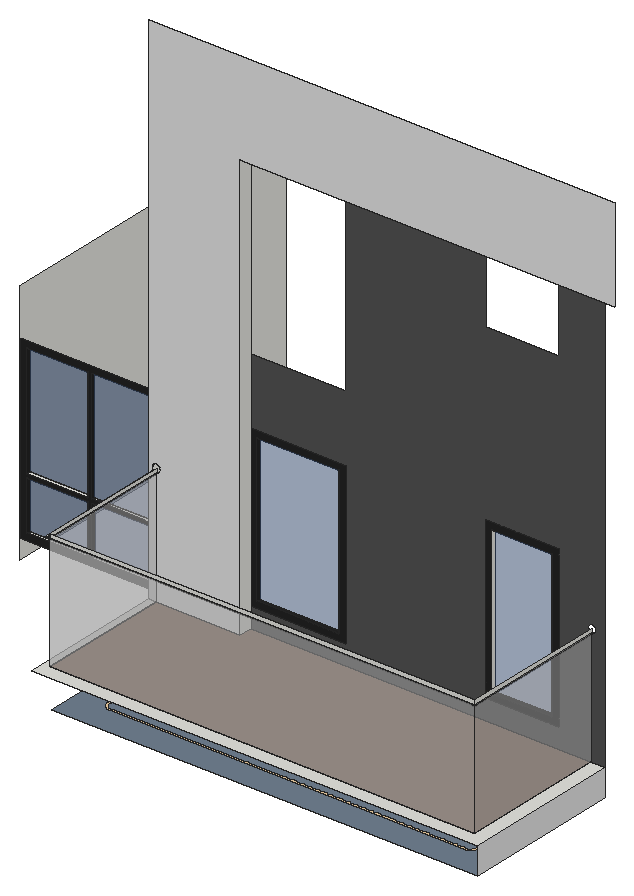
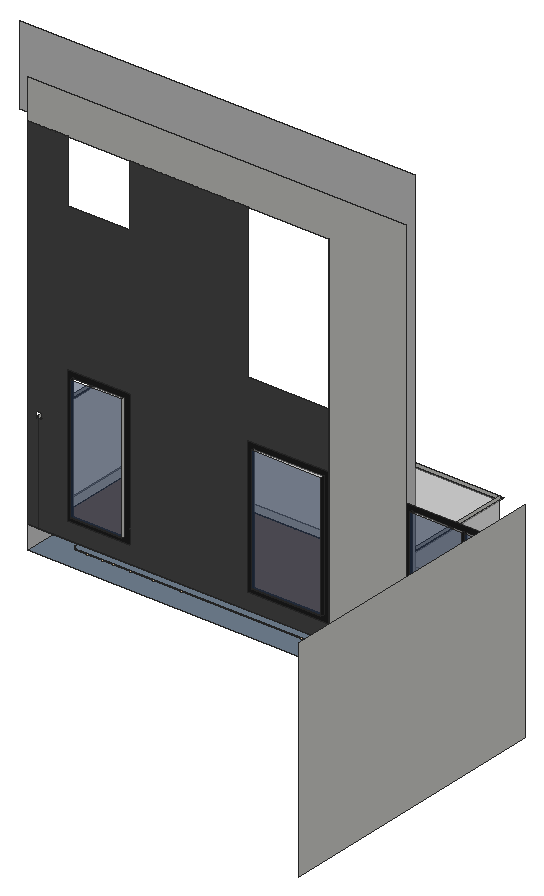
# SketchUp Ruby script. Lengths in inches.
U = 1.inch
M = Sketchup.active_model
def pt(a) = Geom::Point3d.new(a.map { |v| v * U })
def face(e, loops, mat)
  f = e.add_face(loops[0].map { |a| pt(a) })
  loops[1..].each { |l| e.add_face(l.map { |a| pt(a) }).erase! }
  f.material = f.back_material = mat if mat
  f
end
# faces: each face lists its corners as indices into pts; further lists are holes
def faces(e, pts, list, mat = nil) = list.each { |f| face(e, (f[0].is_a?(Array) ? f : [f]).map { |l| l.map { |i| pts[i] } }, mat) }
# xy, xz, yz: faces in a plane at the given z, y or x. An outline is a flat list of corners, or four numbers for a rectangle; further outlines are holes
def ring(l) = l.size == 4 ? [[l[0], l[1]], [l[2], l[1]], [l[2], l[3]], [l[0], l[3]]] : l.each_slice(2).to_a
def flat(e, list, mat, &to3) = list.each { |f| face(e, (f[0].is_a?(Array) ? f : [f]).map { |l| ring(l).map { |u, v| to3.(u, v) } }, mat) }
def xy(e, z, list, mat = nil) = flat(e, list, mat) { |x, y| [x, y, z] }
def xz(e, y, list, mat = nil) = flat(e, list, mat) { |x, z| [x, y, z] }
def yz(e, x, list, mat = nil) = flat(e, list, mat) { |y, z| [x, y, z] }
def lines(e, pts, list) = list.each { |a, b| e.add_line(pt(pts[a]), pt(pts[b])) }
# prism: a flat outline (further loops are holes) pulled along v
def prism(e, loops, v, mat = nil)
  f = face(e, loops, mat); d = Geom::Vector3d.new(v.map { |x| x * U })
  f.pushpull(f.normal.samedirection?(d) ? d.length : -d.length)
end
def box(e, o, s, mat = nil) = prism(e, [[o, [o[0] + s[0], o[1], o[2]], [o[0] + s[0], o[1] + s[1], o[2]], [o[0], o[1] + s[1], o[2]]]], [0, 0, s[2]], mat)
def at(x, y, z, deg = 0) = Geom::Transformation.translation(pt([x, y, z])) * Geom::Transformation.rotation(ORIGIN, Z_AXIS, deg.degrees)
def axes(o, x, y, z) = Geom::Transformation.new([*x, 0, *y, 0, *z, 0, *pt(o).to_a, 1])
def part(name) = M.definitions.add(name)
# library, detail: a bought-in or finely detailed component or shape, given as its bounding box
def library(name, o, s) = part(name).tap { |d| box(d.entities, o, s) }
def detail(e, o, s) = box(e.add_group.entities, o, s)
def put(e, d, t, mat = nil) = e.add_instance(d, t).tap { |i| i.material = mat if mat }
def group(e, t, mat = nil) = e.add_group.tap { |g| g.transformation = t; g.material = mat if mat }.entities
root = M.entities
M.materials.add("[0033_NavajoWhite]1").color = [237, 206, 160]
M.materials.add("[0111_SlateGray]").color = [112, 128, 144]
M.materials.add("[0136_Charcoal]").color = [35, 35, 35]
M.materials.add("[Cladding Siding White]1").color = [224, 224, 224]
M.materials.add("[Cladding Siding White]2").color = [81, 81, 81]
M.materials.add("[Granite Brown]").color = [126, 104, 91]
M.materials.add("[Translucent Glass Blue]").color = [52, 78, 124]
M.materials["[Translucent Glass Blue]"].alpha = 0.5
M.materials.add("[Translucent Glass Gray]").color = [211, 211, 211]
M.materials["[Translucent Glass Gray]"].alpha = 0.5
xy(root,1366.34,[[[412.89,49.29,410.86,49.43,408.86,49.83,406.92,50.48,405.09,51.38,403.4,52.52,401.86,53.86,400.52,55.4,399.38,57.09,398.48,58.92,397.83,60.86,397.43,62.86,397.29,64.89,397.29,223.11,397.43,225.14,397.83,227.14,398.48,229.08,399.38,230.91,400.52,232.6,401.86,234.14,403.4,235.48,405.09,236.62,406.92,237.52,408.86,238.17,410.86,238.57,412.89,238.71,1051.11,238.71,1053.14,238.57,1055.14,238.17,1057.08,237.52,1058.91,236.62,1060.6,235.48,1062.14,234.14,1063.48,232.6,1064.62,230.91,1065.52,229.08,1066.17,227.14,1066.57,225.14,1066.71,223.11,1066.71,64.89,1066.57,62.86,1066.17,60.86,1065.52,58.92,1064.62,57.09,1063.48,55.4,1062.14,53.86,1060.6,52.52,1058.91,51.38,1057.08,50.48,1055.14,49.83,1053.14,49.43,1051.11,49.29],[412.89,53.53,1051.11,53.53,1052.59,53.625,1054.05,53.92,1055.45,54.39,1056.79,55.05,1058.02,55.88,1059.14,56.86,1060.12,57.98,1060.95,59.21,1061.61,60.55,1062.08,61.95,1062.375,63.41,1062.47,64.89,1062.47,223.11,1062.375,224.59,1062.08,226.05,1061.61,227.45,1060.95,228.79,1060.12,230.02,1059.14,231.14,1058.02,232.12,1056.79,232.95,1055.45,233.61,1054.05,234.08,1052.59,234.375,1051.11,234.47,412.89,234.47,411.41,234.375,409.95,234.08,408.55,233.61,407.21,232.95,405.98,232.12,404.86,231.14,403.88,230.02,403.05,228.79,402.39,227.45,401.92,226.05,401.625,224.59,401.53,223.11,401.53,64.89,401.625,63.41,401.92,61.95,402.39,60.55,403.05,59.21,403.88,57.98,404.86,56.86,405.98,55.88,407.21,55.05,408.55,54.39,409.95,53.92,411.41,53.625]]],"[0033_NavajoWhite]1")
xy(root,1366.34,[[[348,0,1116,288],[412.89,49.29,1051.11,49.29,1053.14,49.43,1055.14,49.83,1057.08,50.48,1058.91,51.38,1060.6,52.52,1062.14,53.86,1063.48,55.4,1064.62,57.09,1065.52,58.92,1066.17,60.86,1066.57,62.86,1066.71,64.89,1066.71,223.11,1066.57,225.14,1066.17,227.14,1065.52,229.08,1064.62,230.91,1063.48,232.6,1062.14,234.14,1060.6,235.48,1058.91,236.62,1057.08,237.52,1055.14,238.17,1053.14,238.57,1051.11,238.71,412.89,238.71,410.86,238.57,408.86,238.17,406.92,237.52,405.09,236.62,403.4,235.48,401.86,234.14,400.52,232.6,399.38,230.91,398.48,229.08,397.83,227.14,397.43,225.14,397.29,223.11,397.29,64.89,397.43,62.86,397.83,60.86,398.48,58.92,399.38,57.09,400.52,55.4,401.86,53.86,403.4,52.52,405.09,51.38,406.92,50.48,408.86,49.83,410.86,49.43]],[[412.89,53.53,411.41,53.625,409.95,53.92,408.55,54.39,407.21,55.05,405.98,55.88,404.86,56.86,403.88,57.98,403.05,59.21,402.39,60.55,401.92,61.95,401.625,63.41,401.53,64.89,401.53,223.11,401.625,224.59,401.92,226.05,402.39,227.45,403.05,228.79,403.88,230.02,404.86,231.14,405.98,232.12,407.21,232.95,408.55,233.61,409.95,234.08,411.41,234.375,412.89,234.47,1051.11,234.47,1052.59,234.375,1054.05,234.08,1055.45,233.61,1056.79,232.95,1058.02,232.12,1059.14,231.14,1060.12,230.02,1060.95,228.79,1061.61,227.45,1062.08,226.05,1062.375,224.59,1062.47,223.11,1062.47,64.89,1062.375,63.41,1062.08,61.95,1061.61,60.55,1060.95,59.21,1060.12,57.98,1059.14,56.86,1058.02,55.88,1056.79,55.05,1055.45,54.39,1054.05,53.92,1052.59,53.625,1051.11,53.53],[535.65,130.71,536.9,130.83,538.13,131.08,539.33,131.46,540.48,131.96,541.58,132.58,542.6,133.32,543.54,134.15,544.38,135.08,545.13,136.09,545.77,137.17,546.29,138.3125,546.68,139.5,546.95,140.73,547.09,141.98,547.1,143.24,546.98,144.49,546.73,145.72,546.35,146.91,545.85,148.06,545.23,149.16,544.5,150.18,543.66,151.12,542.74,151.97,541.73,152.71,540.64,153.35,539.5,153.87,538.31,154.26,537.08,154.54,535.83,154.68,534.58,154.6875,533.33,154.5625,532.1,154.3125,530.9,153.93,529.75,153.43,528.66,152.8125,527.63,152.08,526.69,151.25,525.85,150.32,525.1,149.31,524.47,148.23,523.95,147.08,523.55,145.89,523.28,144.66,523.14,143.42,523.13,142.16,523.25,140.91,523.5,139.68,523.88,138.48,524.38,137.33,525,136.24,525.73,135.22,526.57,134.28,527.49,133.43,528.5,132.68,529.59,132.05,530.73,131.53,531.92,131.13,533.15,130.86,534.4,130.72],[899.19,130.71,900.44,130.83,901.67,131.08,902.86,131.46,904.01,131.96,905.11,132.58,906.13,133.32,907.07,134.15,907.92,135.08,908.66,136.09,909.3,137.17,909.82,138.3125,910.21,139.5,910.49,140.73,910.625,141.98,910.64,143.24,910.51,144.49,910.26,145.72,909.88,146.91,909.38,148.06,908.76,149.16,908.03,150.18,907.2,151.12,906.27,151.97,905.26,152.71,904.18,153.35,903.03,153.87,901.84,154.26,900.61,154.54,899.37,154.68,898.11,154.6875,896.86,154.5625,895.63,154.3125,894.43,153.93,893.28,153.43,892.1875,152.8125,891.17,152.08,890.23,151.25,889.38,150.32,888.63,149.31,888,148.23,887.48,147.08,887.08,145.89,886.81,144.66,886.67,143.42,886.66,142.16,886.78,140.91,887.03,139.68,887.41,138.48,887.91,137.33,888.53,136.24,889.27,135.22,890.1,134.28,891.03,133.43,892.04,132.68,893.12,132.05,894.26,131.53,895.45,131.13,896.68,130.86,897.93,130.72]]],"[0111_SlateGray]")
xy(root,1367.34,[[535.65,130.71,534.4,130.72,533.15,130.86,531.92,131.13,530.73,131.53,529.59,132.05,528.5,132.68,527.49,133.43,526.57,134.28,525.73,135.22,525,136.24,524.38,137.33,523.88,138.48,523.5,139.68,523.25,140.91,523.13,142.16,523.14,143.42,523.28,144.66,523.55,145.89,523.95,147.08,524.47,148.23,525.1,149.31,525.85,150.32,526.69,151.25,527.63,152.08,528.66,152.8125,529.75,153.43,530.9,153.93,532.1,154.3125,533.33,154.5625,534.58,154.6875,535.83,154.68,537.08,154.54,538.31,154.26,539.5,153.87,540.64,153.35,541.73,152.71,542.74,151.97,543.66,151.12,544.5,150.18,545.23,149.16,545.85,148.06,546.35,146.91,546.73,145.72,546.98,144.49,547.1,143.24,547.09,141.98,546.95,140.73,546.68,139.5,546.29,138.3125,545.77,137.17,545.13,136.09,544.38,135.08,543.54,134.15,542.6,133.32,541.58,132.58,540.48,131.96,539.33,131.46,538.13,131.08,536.9,130.83],[899.19,130.71,897.93,130.72,896.68,130.86,895.45,131.13,894.26,131.53,893.12,132.05,892.04,132.68,891.03,133.43,890.1,134.28,889.27,135.22,888.53,136.24,887.91,137.33,887.41,138.48,887.03,139.68,886.78,140.91,886.66,142.16,886.67,143.42,886.81,144.66,887.08,145.89,887.48,147.08,888,148.23,888.63,149.31,889.38,150.32,890.23,151.25,891.17,152.08,892.1875,152.8125,893.28,153.43,894.43,153.93,895.63,154.3125,896.86,154.5625,898.11,154.6875,899.37,154.68,900.61,154.54,901.84,154.26,903.03,153.87,904.18,153.35,905.26,152.71,906.27,151.97,907.2,151.12,908.03,150.18,908.76,149.16,909.38,148.06,909.88,146.91,910.26,145.72,910.51,144.49,910.64,143.24,910.625,141.98,910.49,140.73,910.21,139.5,909.82,138.3125,909.3,137.17,908.66,136.09,907.92,135.08,907.07,134.15,906.13,133.32,905.11,132.58,904.01,131.96,902.86,131.46,901.67,131.08,900.44,130.83]])
xy(root,1416,[[312,0,1116,0,1116,288,1092.15,288,1092.15,24,325.23,24,325.23,264,312,264]])
xy(root,1416,[[325.23,24,1092.15,24,1092.15,288,475.9375,288,475.9375,264,325.23,264]],"[Granite Brown]")
xy(root,1428,[[72,288,183,294],[189,288,300,295]])
xy(root,1464,[[487.9375,288,636,294],[912,288,1020,294]],"[0136_Charcoal]")
xy(root,1518,[[72,288,183,294],[189,288,300,295]],"[0136_Charcoal]")
xy(root,1524,[[72,288,183,294],[189,288,300,294]])
xz(root,24,[[325.23,1625,1092.15,1632]])
xz(root,24,[[325.23,1416,1092.15,1625]],"[Translucent Glass Gray]")
xz(root,264,[[325.23,1625,324.5,1625.04,323.78,1625.15,323.07,1625.34,322.39,1625.61,321.73,1625.9375,321.12,1626.34,320.55,1626.8,320.03,1627.32,319.57,1627.89,319.17,1628.5,318.84,1629.15,318.58,1629.84,318.39,1630.54,318.27,1631.27,318.23,1632,318.27,1632.73,318.39,1633.46,318.58,1634.16,318.84,1634.85,319.17,1635.5,319.57,1636.11,320.03,1636.68,320.55,1637.2,321.12,1637.66,321.73,1638.0625,322.39,1638.39,323.07,1638.66,323.78,1638.85,324.5,1638.96,325.23,1639,325.96,1638.96,326.6875,1638.85,327.4,1638.66,328.08,1638.39,328.73,1638.0625,329.35,1637.66,329.92,1637.2,330.43,1636.68,330.9,1636.11,331.29,1635.5,331.63,1634.85,331.89,1634.16,332.08,1633.46,332.19,1632.73,332.23,1632,332.19,1631.27,332.08,1630.54,331.89,1629.84,331.63,1629.15,331.29,1628.5,330.9,1627.89,330.43,1627.32,329.92,1626.8,329.35,1626.34,328.73,1625.9375,328.08,1625.61,327.4,1625.34,326.6875,1625.15,325.96,1625.04]])
xz(root,264,[[[312,1416,475.9375,1416,475.9375,2184,1152,2184,1152,2352,312,2352],[325.23,1625,324.5,1625.04,323.78,1625.15,323.07,1625.34,322.39,1625.61,321.73,1625.9375,321.12,1626.34,320.55,1626.8,320.03,1627.32,319.57,1627.89,319.17,1628.5,318.84,1629.15,318.58,1629.84,318.39,1630.54,318.27,1631.27,318.23,1632,318.27,1632.73,318.39,1633.46,318.58,1634.16,318.84,1634.85,319.17,1635.5,319.57,1636.11,320.03,1636.68,320.55,1637.2,321.12,1637.66,321.73,1638.0625,322.39,1638.39,323.07,1638.66,323.78,1638.85,324.5,1638.96,325.23,1639,325.96,1638.96,326.6875,1638.85,327.4,1638.66,328.08,1638.39,328.73,1638.0625,329.35,1637.66,329.92,1637.2,330.43,1636.68,330.9,1636.11,331.29,1635.5,331.63,1634.85,331.89,1634.16,332.08,1633.46,332.19,1632.73,332.23,1632,332.19,1631.27,332.08,1630.54,331.89,1629.84,331.63,1629.15,331.29,1628.5,330.9,1627.89,330.43,1627.32,329.92,1626.8,329.35,1626.34,328.73,1625.9375,328.08,1625.61,327.4,1625.34,326.6875,1625.15,325.96,1625.04]]],"[Cladding Siding White]1")
xz(root,288,[[312,1416,312,2268,1116,2268,1116,2184,475.9375,2184,475.9375,1416]])
xz(root,288,[[[60,1416,312,1740],[189,1524,300,1728],[72,1524,183,1728],[72,1428,72,1518,183,1518,183,1428,189,1428,189,1518,300,1518,300,1428]],[[475.9375,1452,648,1740],[487.9375,1464,636,1728]],[[900,1452,1032,1740],[912,1464,1020,1728]]],"[0136_Charcoal]")
xz(root,288,[[[475.9375,1416,1116,1416,1116,2184,1032,2184,1032,2052,900,2052,900,2184,648,2184,648,1860,475.9375,1860,475.9375,1740,648,1740,648,1452,475.9375,1452],[900,1452,1032,1740],[1092.15,1625,1091.41,1625.04,1090.69,1625.15,1089.98,1625.34,1089.3,1625.61,1088.65,1625.9375,1088.03,1626.34,1087.46,1626.8,1086.94,1627.32,1086.48,1627.89,1086.08,1628.5,1085.75,1629.15,1085.49,1629.84,1085.3,1630.54,1085.18,1631.27,1085.15,1632,1085.18,1632.73,1085.3,1633.46,1085.49,1634.16,1085.75,1634.85,1086.08,1635.5,1086.48,1636.11,1086.94,1636.68,1087.46,1637.2,1088.03,1637.66,1088.65,1638.0625,1089.3,1638.39,1089.98,1638.66,1090.69,1638.85,1091.41,1638.96,1092.15,1639,1092.88,1638.96,1093.6,1638.85,1094.31,1638.66,1094.99,1638.39,1095.65,1638.0625,1096.26,1637.66,1096.83,1637.2,1097.35,1636.68,1097.81,1636.11,1098.21,1635.5,1098.54,1634.85,1098.8,1634.16,1098.99,1633.46,1099.11,1632.73,1099.15,1632,1099.11,1631.27,1098.99,1630.54,1098.8,1629.84,1098.54,1629.15,1098.21,1628.5,1097.81,1627.89,1097.35,1627.32,1096.83,1626.8,1096.26,1626.34,1095.65,1625.9375,1094.99,1625.61,1094.31,1625.34,1093.6,1625.15,1092.88,1625.04]]],"[Cladding Siding White]2")
xz(root,294,[[72,1428,183,1518],[487.9375,1464,636,1728],[912,1464,1020,1728],[72,1524,183,1728],[189,1524,300,1728]],"[Translucent Glass Blue]")
xz(root,295,[[189,1428,300,1518]],"[Translucent Glass Blue]")
yz(root,60,[[288,1380,888,1824]])
yz(root,72,[[288,1428,294,1518],[288,1524,294,1728]],"[0136_Charcoal]")
yz(root,183,[[288,1428,294,1518]])
yz(root,183,[[288,1524,294,1728]],"[0136_Charcoal]")
yz(root,189,[[288,1428,295,1518],[288,1524,294,1728]],"[0136_Charcoal]")
yz(root,300,[[288,1428,295,1518],[288,1524,294,1728]],"[0136_Charcoal]")
yz(root,325.23,[[24,1625,264,1632]])
yz(root,325.23,[[24,1416,264,1625]],"[Translucent Glass Gray]")
yz(root,475.9375,[[264,1416,288,2184]])
yz(root,487.9375,[[288,1464,294,1728]],"[0136_Charcoal]")
yz(root,636,[[288,1464,294,1728]],"[0136_Charcoal]")
yz(root,912,[[288,1464,294,1728]])
yz(root,1020,[[288,1464,294,1728]],"[0136_Charcoal]")
yz(root,1092.15,[[24,1625,288,1632]])
yz(root,1092.15,[[24,1416,288,1625]],"[Translucent Glass Gray]")
yz(root,1116,[[0,1366.34,288,1416]],"[Cladding Siding White]1")
p = [[534.4,130.72,1366.34],[533.15,130.86,1366.34],[533.15,130.86,1367.34],[534.4,130.72,1367.34],[535.65,130.71,1366.34],[535.65,130.71,1367.34],
  [536.9,130.83,1366.34],[536.9,130.83,1367.34],[897.93,130.72,1366.34],[896.68,130.86,1366.34],[896.68,130.86,1367.34],[897.93,130.72,1367.34],
  [899.19,130.71,1366.34],[899.19,130.71,1367.34],[900.44,130.83,1366.34],[900.44,130.83,1367.34],[538.13,131.08,1366.34],[538.13,131.08,1367.34],
  [901.67,131.08,1366.34],[901.67,131.08,1367.34],[531.92,131.13,1366.34],[531.92,131.13,1367.34],[895.45,131.13,1366.34],[895.45,131.13,1367.34],
  [530.73,131.53,1366.34],[530.73,131.53,1367.34],[539.33,131.46,1366.34],[539.33,131.46,1367.34],[894.26,131.53,1366.34],[894.26,131.53,1367.34],
  [902.86,131.46,1366.34],[902.86,131.46,1367.34],[529.59,132.05,1366.34],[529.59,132.05,1367.34],[540.48,131.96,1366.34],[540.48,131.96,1367.34],
  [893.12,132.05,1366.34],[893.12,132.05,1367.34],[904.01,131.96,1366.34],[904.01,131.96,1367.34],[528.5,132.68,1366.34],[528.5,132.68,1367.34],
  [541.58,132.58,1366.34],[541.58,132.58,1367.34],[892.04,132.68,1366.34],[892.04,132.68,1367.34],[905.11,132.58,1366.34],[905.11,132.58,1367.34],
  [542.6,133.32,1366.34],[542.6,133.32,1367.34],[906.13,133.32,1366.34],[906.13,133.32,1367.34],[527.49,133.43,1366.34],[527.49,133.43,1367.34],
  [891.03,133.43,1366.34],[891.03,133.43,1367.34],[543.54,134.15,1366.34],[543.54,134.15,1367.34],[907.07,134.15,1366.34],[907.07,134.15,1367.34],
  [526.57,134.28,1366.34],[526.57,134.28,1367.34],[890.1,134.28,1366.34],[890.1,134.28,1367.34],[544.38,135.08,1366.34],[544.38,135.08,1367.34],
  [907.92,135.08,1366.34],[907.92,135.08,1367.34],[525.73,135.22,1366.34],[525.73,135.22,1367.34],[889.27,135.22,1366.34],[889.27,135.22,1367.34],
  [545.13,136.09,1366.34],[545.13,136.09,1367.34],[908.66,136.09,1366.34],[908.66,136.09,1367.34],[525,136.24,1366.34],[525,136.24,1367.34],
  [888.53,136.24,1366.34],[888.53,136.24,1367.34],[545.77,137.17,1366.34],[545.77,137.17,1367.34],[909.3,137.17,1366.34],[909.3,137.17,1367.34],
  [524.38,137.33,1366.34],[524.38,137.33,1367.34],[887.91,137.33,1366.34],[887.91,137.33,1367.34],[546.29,138.3125,1366.34],[546.29,138.3125,1367.34],
  [909.82,138.3125,1366.34],[909.82,138.3125,1367.34],[523.88,138.48,1366.34],[523.88,138.48,1367.34],[887.41,138.48,1366.34],[887.41,138.48,1367.34],
  [546.68,139.5,1366.34],[546.68,139.5,1367.34],[910.21,139.5,1366.34],[910.21,139.5,1367.34],[523.5,139.68,1366.34],[523.5,139.68,1367.34],
  [887.03,139.68,1366.34],[887.03,139.68,1367.34],[546.95,140.73,1366.34],[546.95,140.73,1367.34],[910.49,140.73,1366.34],[910.49,140.73,1367.34],
  [523.25,140.91,1366.34],[523.25,140.91,1367.34],[886.78,140.91,1366.34],[886.78,140.91,1367.34],[547.09,141.98,1366.34],[547.09,141.98,1367.34],
  [910.625,141.98,1366.34],[910.625,141.98,1367.34],[523.13,142.16,1366.34],[523.13,142.16,1367.34],[886.66,142.16,1366.34],[886.66,142.16,1367.34],
  [547.1,143.24,1366.34],[547.1,143.24,1367.34],[910.64,143.24,1366.34],[910.64,143.24,1367.34],[523.14,143.42,1366.34],[523.14,143.42,1367.34],
  [886.67,143.42,1366.34],[886.67,143.42,1367.34],[546.98,144.49,1366.34],[546.98,144.49,1367.34],[910.51,144.49,1366.34],[910.51,144.49,1367.34],
  [523.28,144.66,1366.34],[523.28,144.66,1367.34],[886.81,144.66,1366.34],[886.81,144.66,1367.34],[546.73,145.72,1366.34],[546.73,145.72,1367.34],
  [910.26,145.72,1366.34],[910.26,145.72,1367.34],[523.55,145.89,1366.34],[523.55,145.89,1367.34],[887.08,145.89,1366.34],[887.08,145.89,1367.34],
  [546.35,146.91,1366.34],[546.35,146.91,1367.34],[909.88,146.91,1366.34],[909.88,146.91,1367.34],[523.95,147.08,1366.34],[523.95,147.08,1367.34],
  [887.48,147.08,1366.34],[887.48,147.08,1367.34],[545.85,148.06,1366.34],[545.85,148.06,1367.34],[909.38,148.06,1366.34],[909.38,148.06,1367.34],
  [524.47,148.23,1366.34],[524.47,148.23,1367.34],[888,148.23,1366.34],[888,148.23,1367.34],[545.23,149.16,1366.34],[545.23,149.16,1367.34],
  [908.76,149.16,1366.34],[908.76,149.16,1367.34],[525.1,149.31,1366.34],[525.1,149.31,1367.34],[888.63,149.31,1366.34],[888.63,149.31,1367.34],
  [544.5,150.18,1366.34],[544.5,150.18,1367.34],[908.03,150.18,1366.34],[908.03,150.18,1367.34],[525.85,150.32,1366.34],[525.85,150.32,1367.34],
  [889.38,150.32,1366.34],[889.38,150.32,1367.34],[543.66,151.12,1366.34],[543.66,151.12,1367.34],[907.2,151.12,1366.34],[907.2,151.12,1367.34],
  [526.69,151.25,1366.34],[526.69,151.25,1367.34],[890.23,151.25,1366.34],[890.23,151.25,1367.34],[542.74,151.97,1366.34],[542.74,151.97,1367.34],
  [906.27,151.97,1366.34],[906.27,151.97,1367.34],[527.63,152.08,1366.34],[527.63,152.08,1367.34],[891.17,152.08,1366.34],[891.17,152.08,1367.34],
  [541.73,152.71,1366.34],[541.73,152.71,1367.34],[905.26,152.71,1366.34],[905.26,152.71,1367.34],[528.66,152.8125,1366.34],[528.66,152.8125,1367.34],
  [892.1875,152.8125,1366.34],[892.1875,152.8125,1367.34],[540.64,153.35,1366.34],[540.64,153.35,1367.34],[904.18,153.35,1366.34],[904.18,153.35,1367.34],
  [529.75,153.43,1366.34],[529.75,153.43,1367.34],[893.28,153.43,1366.34],[893.28,153.43,1367.34],[539.5,153.87,1366.34],[539.5,153.87,1367.34],
  [903.03,153.87,1366.34],[903.03,153.87,1367.34],[530.9,153.93,1366.34],[530.9,153.93,1367.34],[894.43,153.93,1366.34],[894.43,153.93,1367.34],
  [532.1,154.3125,1366.34],[532.1,154.3125,1367.34],[538.31,154.26,1366.34],[538.31,154.26,1367.34],[895.63,154.3125,1366.34],[895.63,154.3125,1367.34],
  [901.84,154.26,1366.34],[901.84,154.26,1367.34],[533.33,154.5625,1366.34],[533.33,154.5625,1367.34],[537.08,154.54,1366.34],[537.08,154.54,1367.34],
  [896.86,154.5625,1366.34],[896.86,154.5625,1367.34],[900.61,154.54,1366.34],[900.61,154.54,1367.34],[535.83,154.68,1366.34],[535.83,154.68,1367.34],
  [899.37,154.68,1366.34],[899.37,154.68,1367.34],[534.58,154.6875,1366.34],[534.58,154.6875,1367.34],[898.11,154.6875,1366.34],[898.11,154.6875,1367.34],
  [323.78,264,1625.15],[324.5,264,1625.04],[324.5,23.27,1625.04],[323.78,22.54,1625.15],[1092.88,23.27,1625.04],[1093.6,22.54,1625.15],
  [1092.88,288,1625.04],[1093.6,288,1625.15],[325.23,264,1625],[325.23,24,1625],[1092.15,24,1625],[1092.15,288,1625],
  [325.96,264,1625.04],[325.96,24.73,1625.04],[1091.41,24.73,1625.04],[1091.41,288,1625.04],[326.6875,264,1625.15],[326.6875,25.46,1625.15],
  [1090.69,25.46,1625.15],[1090.69,288,1625.15],[323.07,264,1625.34],[323.07,21.84,1625.34],[1094.31,21.84,1625.34],[1094.31,288,1625.34],
  [327.4,264,1625.34],[327.4,26.16,1625.34],[1089.98,26.16,1625.34],[1089.98,288,1625.34],[322.39,264,1625.61],[322.39,21.15,1625.61],
  [1094.99,21.15,1625.61],[1094.99,288,1625.61],[328.08,264,1625.61],[328.08,26.85,1625.61],[1089.3,26.85,1625.61],[1089.3,288,1625.61],
  [321.73,264,1625.9375],[321.73,20.5,1625.9375],[1095.65,20.5,1625.9375],[1095.65,288,1625.9375],[328.73,264,1625.9375],[328.73,27.5,1625.9375],
  [1088.65,27.5,1625.9375],[1088.65,288,1625.9375],[321.12,264,1626.34],[321.12,19.89,1626.34],[1096.26,19.89,1626.34],[1096.26,288,1626.34],
  [329.35,264,1626.34],[329.35,28.11,1626.34],[1088.03,28.11,1626.34],[1088.03,288,1626.34],[320.55,264,1626.8],[320.55,19.32,1626.8],
  [1096.83,19.32,1626.8],[1096.83,288,1626.8],[329.92,264,1626.8],[329.92,28.68,1626.8],[1087.46,28.68,1626.8],[1087.46,288,1626.8],
  [320.03,264,1627.32],[320.03,18.8,1627.32],[1097.35,18.8,1627.32],[1097.35,288,1627.32],[330.43,264,1627.32],[330.43,29.2,1627.32],
  [1086.94,29.2,1627.32],[1086.94,288,1627.32]]
faces(root,p,[[0,1,2,3],[4,0,3,5],[6,4,5,7],[8,9,10,11],[12,8,11,13],[14,12,13,15],[16,6,7,17],[18,14,15,19],
  [1,20,21,2],[9,22,23,10],[20,24,25,21],[26,16,17,27],[22,28,29,23],[30,18,19,31],[24,32,33,25],[34,26,27,35],
  [28,36,37,29],[38,30,31,39],[32,40,41,33],[42,34,35,43],[36,44,45,37],[46,38,39,47],[48,42,43,49],[50,46,47,51],
  [40,52,53,41],[44,54,55,45],[56,48,49,57],[58,50,51,59],[52,60,61,53],[54,62,63,55],[64,56,57,65],[66,58,59,67],
  [60,68,69,61],[62,70,71,63],[72,64,65,73],[74,66,67,75],[68,76,77,69],[70,78,79,71],[80,72,73,81],[82,74,75,83],
  [76,84,85,77],[78,86,87,79],[88,80,81,89],[90,82,83,91],[84,92,93,85],[86,94,95,87],[96,88,89,97],[98,90,91,99],
  [92,100,101,93],[94,102,103,95],[104,96,97,105],[106,98,99,107],[100,108,109,101],[102,110,111,103],[112,104,105,113],[114,106,107,115],
  [108,116,117,109],[110,118,119,111],[120,112,113,121],[122,114,115,123],[116,124,125,117],[118,126,127,119],[128,120,121,129],[130,122,123,131],
  [124,132,133,125],[126,134,135,127],[136,128,129,137],[138,130,131,139],[132,140,141,133],[134,142,143,135],[144,136,137,145],[146,138,139,147],
  [140,148,149,141],[142,150,151,143],[152,144,145,153],[154,146,147,155],[148,156,157,149],[150,158,159,151],[160,152,153,161],[162,154,155,163],
  [156,164,165,157],[158,166,167,159],[168,160,161,169],[170,162,163,171],[164,172,173,165],[166,174,175,167],[176,168,169,177],[178,170,171,179],
  [172,180,181,173],[174,182,183,175],[184,176,177,185],[186,178,179,187],[180,188,189,181],[182,190,191,183],[192,184,185,193],[194,186,187,195],
  [188,196,197,189],[190,198,199,191],[200,192,193,201],[202,194,195,203],[196,204,205,197],[198,206,207,199],[208,200,201,209],[210,202,203,211],
  [204,212,213,205],[206,214,215,207],[212,216,217,213],[218,208,209,219],[214,220,221,215],[222,210,211,223],[216,224,225,217],[226,218,219,227],
  [220,228,229,221],[230,222,223,231],[232,226,227,233],[234,230,231,235],[224,236,237,225],[228,238,239,229],[236,232,233,237],[238,234,235,239],
  [240,241,242,243],[243,242,244,245],[245,244,246,247],[241,248,249,242],[242,249,250,244],[244,250,251,246],[248,252,253,249],[249,253,254,250],
  [250,254,255,251],[252,256,257,253],[253,257,258,254],[254,258,259,255],[260,240,243,261],[261,243,245,262],[262,245,247,263],[256,264,265,257],
  [257,265,266,258],[258,266,267,259],[268,260,261,269],[269,261,262,270],[270,262,263,271],[264,272,273,265],[265,273,274,266],[266,274,275,267],
  [276,268,269,277],[277,269,270,278],[278,270,271,279],[272,280,281,273],[273,281,282,274],[274,282,283,275],[284,276,277,285],[285,277,278,286],
  [286,278,279,287],[280,288,289,281],[281,289,290,282],[282,290,291,283],[292,284,285,293],[293,285,286,294],[294,286,287,295],[288,296,297,289],
  [289,297,298,290],[290,298,299,291],[300,292,293,301],[301,293,294,302],[302,294,295,303],[296,304,305,297],[297,305,306,298],[298,306,307,299]])
